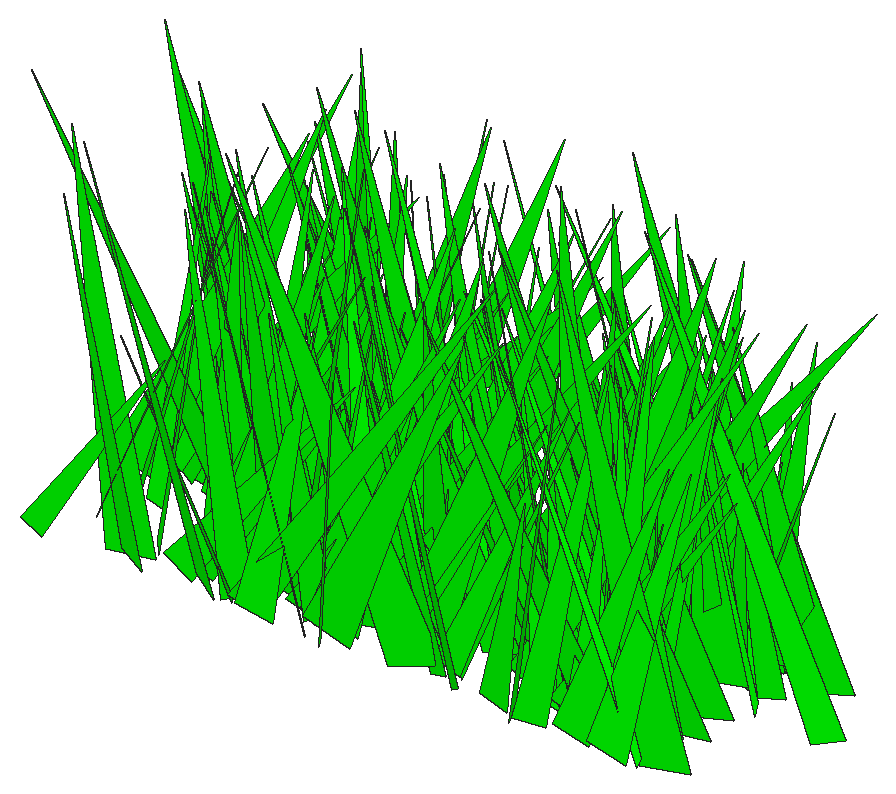
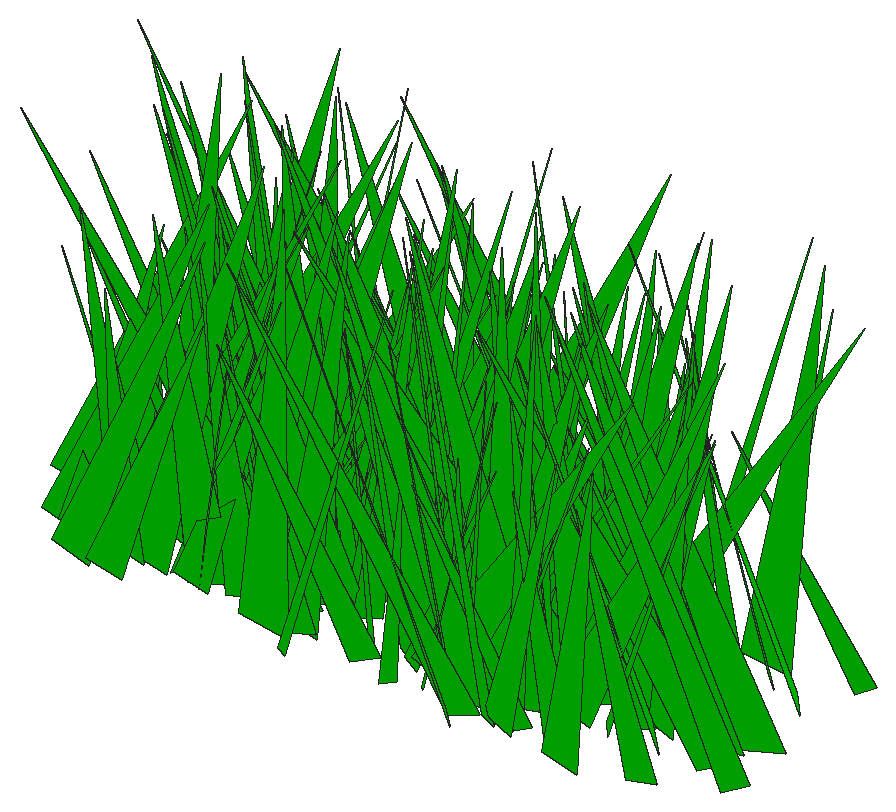
# SketchUp Ruby script. Lengths in inches.
U = 1.inch
M = Sketchup.active_model
def pt(a) = Geom::Point3d.new(a.map { |v| v * U })
def face(e, loops, mat)
  f = e.add_face(loops[0].map { |a| pt(a) })
  loops[1..].each { |l| e.add_face(l.map { |a| pt(a) }).erase! }
  f.material = f.back_material = mat if mat
  f
end
# faces: each face lists its corners as indices into pts; further lists are holes
def faces(e, pts, list, mat = nil) = list.each { |f| face(e, (f[0].is_a?(Array) ? f : [f]).map { |l| l.map { |i| pts[i] } }, mat) }
# xy, xz, yz: faces in a plane at the given z, y or x. An outline is a flat list of corners, or four numbers for a rectangle; further outlines are holes
def ring(l) = l.size == 4 ? [[l[0], l[1]], [l[2], l[1]], [l[2], l[3]], [l[0], l[3]]] : l.each_slice(2).to_a
def flat(e, list, mat, &to3) = list.each { |f| face(e, (f[0].is_a?(Array) ? f : [f]).map { |l| ring(l).map { |u, v| to3.(u, v) } }, mat) }
def xy(e, z, list, mat = nil) = flat(e, list, mat) { |x, y| [x, y, z] }
def xz(e, y, list, mat = nil) = flat(e, list, mat) { |x, z| [x, y, z] }
def yz(e, x, list, mat = nil) = flat(e, list, mat) { |y, z| [x, y, z] }
def lines(e, pts, list) = list.each { |a, b| e.add_line(pt(pts[a]), pt(pts[b])) }
# prism: a flat outline (further loops are holes) pulled along v
def prism(e, loops, v, mat = nil)
  f = face(e, loops, mat); d = Geom::Vector3d.new(v.map { |x| x * U })
  f.pushpull(f.normal.samedirection?(d) ? d.length : -d.length)
end
def box(e, o, s, mat = nil) = prism(e, [[o, [o[0] + s[0], o[1], o[2]], [o[0] + s[0], o[1] + s[1], o[2]], [o[0], o[1] + s[1], o[2]]]], [0, 0, s[2]], mat)
def at(x, y, z, deg = 0) = Geom::Transformation.translation(pt([x, y, z])) * Geom::Transformation.rotation(ORIGIN, Z_AXIS, deg.degrees)
def axes(o, x, y, z) = Geom::Transformation.new([*x, 0, *y, 0, *z, 0, *pt(o).to_a, 1])
def part(name) = M.definitions.add(name)
# library, detail: a bought-in or finely detailed component or shape, given as its bounding box
def library(name, o, s) = part(name).tap { |d| box(d.entities, o, s) }
def detail(e, o, s) = box(e.add_group.entities, o, s)
def put(e, d, t, mat = nil) = e.add_instance(d, t).tap { |i| i.material = mat if mat }
def group(e, t, mat = nil) = e.add_group.tap { |g| g.transformation = t; g.material = mat if mat }.entities
root = M.entities
M.materials.add("[0065_Lime]").color = [0, 255, 0]
c1 = part("fur_instance\#9")
p = [[0.8125,0,1.79],[0.67,-0.02,1.48],[0,-0.11,0],[0,0.11,0]]
faces(c1.entities,p,[[0,1,2,3]])
put(root,c1,axes([68.35,19.12,1.48],[1.92104,-1.04775,2.1483],[7.68559,0.3376,0.9702],[-1.87206,0.31084,6.18757]),"[0065_Lime]")
put(root,c1,axes([69.45,24.6,1.48],[-6.90798,-0.10181,0.94758],[0.97663,-0.95513,1.27214],[0.96343,0.23825,5.50478]),"[0065_Lime]")
put(root,c1,axes([65.31,18.61,1.48],[3.53476,-0.42766,0.80834],[3.08147,0.39799,-1.85976],[0.86889,0.32834,3.30709]),"[0065_Lime]")
put(root,c1,axes([71.52,20.78,1.48],[-6.4799,-0.85162,0.43145],[5.9126,-0.8559,2.14311],[-1.43303,0.31949,6.89142]),"[0065_Lime]")
put(root,c1,axes([68.58,18.88,1.48],[-6.15413,-0.59026,0.7195],[3.89168,-0.85884,-1.58552],[1.81175,-0.16018,5.84974]),"[0065_Lime]")
put(root,c1,axes([64.69,25.02,1.48],[8.06333,-0.48685,0.88652],[3.63083,1.09017,-1.7887],[-0.09462,0.34461,6.91094]),"[0065_Lime]")
put(root,c1,axes([67.125,21.7,1.48],[6.69471,-0.16008,2.11529],[1.84591,0.95655,-1.43968],[-2.15711,0.32173,5.33293]),"[0065_Lime]")
put(root,c1,axes([68.27,23.74,1.48],[6.68983,-0.518,2.03854],[2.93109,0.98966,2.0625],[-3.35842,-0.1681,5.86076]),"[0065_Lime]")
put(root,c1,axes([69.69,23.42,1.48],[2.51525,-1.14828,2.51117],[8.20564,0.4654,1.69312],[-2.99597,0.31066,6.74552]),"[0065_Lime]")
put(root,c1,axes([70.84,24.51,1.48],[-0.91679,0.94632,1.41171],[-6.48248,-0.02719,-2.17456],[-2.51871,-0.27446,5.08288]),"[0065_Lime]")
put(root,c1,axes([66.91,26.29,1.48],[0.68411,-0.6995,0.27313],[4.85295,0.08223,-0.98546],[1.15854,0.06859,3.96665]),"[0065_Lime]")
put(root,c1,axes([69.78,23.02,1.48],[1.5787,0.79457,1.56524],[-5.45357,0.30582,-1.56282],[-2.43637,-0.1697,4.51245]),"[0065_Lime]")
put(root,c1,axes([65.42,22.97,1.48],[1.64409,1.11556,1.21062],[-7.7039,0.15243,2.21546],[2.42736,-0.2718,6.2114]),"[0065_Lime]")
put(root,c1,axes([71.14,24.17,1.48],[-6.88015,0.60712,1.02471],[-4.49889,-0.93646,-1.394],[0.12055,-0.2984,6.4597]),"[0065_Lime]")
put(root,c1,axes([66.4,23.58,1.48],[2.17103,1.16452,0.05617],[-8.14962,0.29815,1.28105],[1.50634,-0.06531,6.84977]),"[0065_Lime]")
put(root,c1,axes([66.27,20.3125,1.48],[8.72768,0.24973,0.46553],[-1.53905,1.17989,-2.11864],[-1.05709,0.34403,6.9282]),"[0065_Lime]")
put(root,c1,axes([68.32,22.84,1.48],[-2.65391,0.63624,0.28444],[-4.09765,-0.36002,1.68903],[1.9578,0.10894,3.92069]),"[0065_Lime]")
put(root,c1,axes([69.28,26.88,1.48],[3.03842,-0.77609,0.00496],[5.27021,0.4077,1.53113],[-1.65206,-0.12678,4.89355]),"[0065_Lime]")
put(root,c1,axes([66.93,23.33,1.48],[6.04871,-0.08994,0.3127],[0.73509,0.7946,-1.74977],[-0.13078,0.30651,4.62782]),"[0065_Lime]")
put(root,c1,axes([71.05,18.95,1.48],[-7.99216,-0.55256,0.60294],[3.62149,-1.09775,-1.9491],[1.7021,-0.25888,6.9781]),"[0065_Lime]")
put(root,c1,axes([67.6,19.81,1.48],[7.73344,0.25591,1.04553],[-1.60675,1.09196,-1.09288],[-1.5451,0.14535,6.36949]),"[0065_Lime]")
put(root,c1,axes([68.67,19.9,1.48],[6.51938,0.05109,1.60015],[-0.98298,0.9025,1.68429],[-1.74236,-0.31801,5.03705]),"[0065_Lime]")
put(root,c1,axes([71.42,22.46,1.48],[-6.31564,0.04592,1.05792],[-0.77244,-0.84383,-1.82383],[1.0962,-0.33006,4.80992]),"[0065_Lime]")
put(root,c1,axes([65.83,24.31,1.48],[2.96567,-0.96311,2.07533],[6.5619,0.17958,-3.41155],[3.22936,0.51956,5.02623]),"[0065_Lime]")
put(root,c1,axes([72.04,18.87,1.48],[-4.76381,-0.07754,0.04405],[0.53477,-0.62519,1.38992],[-0.14635,0.23935,3.64483]),"[0065_Lime]")
put(root,c1,axes([68.16,24.125,1.48],[8.31635,0.34784,0.41406],[-1.83086,0.99882,-3.78665],[-1.7421,0.61082,5.95617]),"[0065_Lime]")
put(root,c1,axes([71.09,22.15,1.48],[4.51504,-0.51168,1.58684],[2.68172,0.67193,2.21171],[-3.14226,-0.16176,4.16766]),"[0065_Lime]")
put(root,c1,axes([69.64,21.49,1.48],[4.00086,-0.84633,0.32961],[5.91729,0.56335,0.94841],[-1.19401,-0.04399,5.80456]),"[0065_Lime]")
put(root,c1,axes([70.95,21.35,1.48],[3.66518,-0.68356,1.26875],[4.55252,0.55943,1.39824],[-2.31767,0.01789,4.75292]),"[0065_Lime]")
put(root,c1,axes([69.84,26.12,1.48],[-1.64757,0.6869,0.50919],[-4.71122,-0.24675,1.06789],[1.44657,-0.02126,4.05788]),"[0065_Lime]")
put(root,c1,axes([68.7,23.97,1.48],[1.69245,-0.55072,0.35965],[3.72898,0.20141,-1.27586],[1.28467,0.1409,3.2296]),"[0065_Lime]")
put(root,c1,axes([72.42,25.84,1.48],[-6.50528,0.12939,0.54173],[-0.73196,-0.89306,1.3321],[0.86931,0.21632,5.17554]),"[0065_Lime]")
put(root,c1,axes([72.18,21.05,1.48],[-1.928,0.8871,0.54164],[-6.2842,-0.25287,-0.92229],[-0.89832,-0.13493,5.28946]),"[0065_Lime]")
put(root,c1,axes([72.48,21.85,1.48],[1.47372,-1.19502,2.04646],[8.45244,0.29776,1.79908],[-2.68522,0.28143,6.78624]),"[0065_Lime]")
put(root,c1,axes([71.92,26.26,1.48],[2.7078,0.70632,1.50407],[-4.70658,0.45276,-1.51826],[-2.55605,-0.08543,4.389]),"[0065_Lime]")
put(root,c1,axes([74.25,23.12,1.48],[-7.71029,-0.19198,0.01805],[1.32148,-1.04311,1.71851],[-0.34759,0.29284,6.13314]),"[0065_Lime]")
put(root,c1,axes([70.29,25.74,1.48],[5.65626,-0.02285,1.46593],[-0.45932,0.78575,1.5831],[-1.75026,-0.28006,4.32196]),"[0065_Lime]")
put(root,c1,axes([70.67,23.84,1.48],[-4.0635,1.0657,0.05312],[-7.21549,-0.54641,2.12905],[2.33658,0.166,6.667]),"[0065_Lime]")
put(root,c1,axes([71.875,25.63,1.48],[-7.92677,0.41326,1.77235],[-2.31868,-1.13207,1.98389],[2.8321,0.22984,6.58486]),"[0065_Lime]")
put(root,c1,axes([73.02,21.12,1.48],[3.16708,1.01763,1.30581],[-6.65811,0.49812,-2.32321],[-3.27003,-0.02862,5.99499]),"[0065_Lime]")
put(root,c1,axes([74.93,25.21,1.48],[-1.93715,1.02369,1.59701],[-6.90012,-0.12514,-2.84992],[-3.05223,-0.36681,5.42919]),"[0065_Lime]")
put(root,c1,axes([72.08,19.09,1.48],[5.66412,-0.74574,1.59581],[4.6379,0.83536,2.18939],[-3.24103,-0.10788,5.9219]),"[0065_Lime]")
put(root,c1,axes([70.9,21.29,1.48],[4.70565,0.94097,0.2014],[-6.54395,0.65444,-1.29456],[-1.4424,0.10071,6.53028]),"[0065_Lime]")
put(root,c1,axes([73.21,24.91,1.48],[0.7733,-0.99854,1.88814],[7.20933,0.18636,1.34888],[-1.97758,0.28891,5.65571]),"[0065_Lime]")
put(root,c1,axes([73.92,24.13,1.48],[-0.82948,0.90279,0.70334],[-6.23358,-0.07745,-1.53302],[-1.77981,-0.1495,5.04143]),"[0065_Lime]")
put(root,c1,axes([73.375,21.93,1.48],[-6.63662,0.35878,2.4086],[-3.5877,-0.88466,-2.12489],[1.5543,-0.51007,5.3796]),"[0065_Lime]")
put(root,c1,axes([70.17,20.52,1.48],[2.20365,-0.8752,0.96249],[6.22186,0.26476,-1.35797],[1.21703,0.23115,5.19958]),"[0065_Lime]")
put(root,c1,axes([73.4,20.22,1.48],[-3.22956,-0.40288,1.22892],[3.22937,-0.42522,0.94396],[0.27204,0.26495,3.3836]),"[0065_Lime]")
put(root,c1,axes([70.5,22.81,1.48],[2.78458,-0.73543,0.99269],[5.31238,0.34749,-1.2331],[0.81222,0.24851,4.66189]),"[0065_Lime]")
put(root,c1,axes([72.08,24.39,1.48],[-6.10707,-0.95814,1.8294],[6.47072,-0.91426,-1.75312],[3.11153,0.02073,7.2364]),"[0065_Lime]")
put(root,c1,axes([72.49,22.64,1.48],[3.89497,-0.04542,1.67144],[0.933,0.58597,-0.90493],[-1.85914,0.19891,3.04759]),"[0065_Lime]")
put(root,c1,axes([72.81,20.125,1.48],[-3.85919,-0.97664,0.18074],[6.82242,-0.53867,-1.15258],[1.34543,-0.06983,6.36294]),"[0065_Lime]")
put(root,c1,axes([69.85,20.31,1.48],[7.09166,-0.00725,0.1791],[0.08684,0.98359,-0.9409],[-0.20881,0.16284,5.69135]),"[0065_Lime]")
put(root,c1,axes([74.8,18.55,1.48],[-7.96327,-0.0877,1.18804],[0.87811,-1.11739,1.13044],[1.32351,0.21371,6.39819]),"[0065_Lime]")
put(root,c1,axes([71.0625,19.99,1.48],[-2.73714,0.97285,2.80938],[-7.05841,-0.52481,1.53971],[3.16863,-0.32869,5.85666]),"[0065_Lime]")
put(root,c1,axes([69.79,19.34,1.48],[2.344,0.71962,0.65141],[-4.64176,0.23644,2.29856],[2.30701,-0.25543,3.96291]),"[0065_Lime]")
put(root,c1,axes([70.42,19.52,1.48],[3.20885,-0.54333,0.04601],[3.61815,0.41819,-1.47822],[1.36487,0.16879,3.81045]),"[0065_Lime]")
put(root,c1,axes([73.93,25.09,1.48],[5.81947,0.34316,2.17539],[-1.40303,0.86932,-2.11183],[-3.33883,0.23281,4.67904]),"[0065_Lime]")
put(root,c1,axes([72.92,24.8,1.48],[6.17735,-0.92749,0.46797],[6.21349,0.84934,2.13916],[-2.30013,-0.19655,7.03546]),"[0065_Lime]")
put(root,c1,axes([75.03,21.83,1.48],[-6.41239,-0.06113,1.05776],[0.69563,-0.89805,1.05112],[1.18168,0.19695,5.12115]),"[0065_Lime]")
put(root,c1,axes([75.84,21.9,1.48],[1.6713,1.02963,1.78556],[-6.87504,0.34061,-2.3237],[-3.35308,-0.18516,5.65442]),"[0065_Lime]")
put(root,c1,axes([71.23,26.01,1.48],[4.84109,-0.31149,0.09209],[2.18752,0.66308,-0.93091],[0.37604,0.15272,4.22976]),"[0065_Lime]")
put(root,c1,axes([74.76,25.95,1.48],[-5.99326,-0.13007,1.05201],[0.62914,-0.84463,-1.12778],[1.4607,-0.16987,4.80214]),"[0065_Lime]")
put(root,c1,axes([74.01,25.25,1.48],[2.41619,0.64562,0.22273],[-4.40619,0.33701,-1.10842],[-1.33073,0.05639,4.0745]),"[0065_Lime]")
put(root,c1,axes([72.25,26.25,1.48],[8.42095,-0.18217,1.4288],[0.81257,1.17441,1.84883],[-2.0263,-0.28611,6.67925]),"[0065_Lime]")
put(root,c1,axes([72.98,18.65,1.48],[-0.76014,0.81306,1.00619],[-5.76627,-0.14108,0.9379],[1.32657,-0.14737,4.65339]),"[0065_Lime]")
put(root,c1,axes([73.04,22.48,1.48],[5.10116,-0.03509,1.1362],[0.5886,0.71875,-1.00475],[-1.29113,0.18904,4.03099]),"[0065_Lime]")
put(root,c1,axes([73.54,22.78,1.48],[-3.90133,0.9385,1.18099],[-6.45272,-0.58319,1.42587],[2.25332,-0.04517,6.1279]),"[0065_Lime]")
put(root,c1,axes([71.72,25.09,1.48],[3.36956,-1.12389,1.40913],[8.11841,0.42588,-1.46241],[1.03154,0.31948,6.9065]),"[0065_Lime]")
put(root,c1,axes([72.75,21.02,1.48],[8.51135,-0.10725,1.91097],[0.28924,1.21953,1.44115],[-2.45321,-0.22832,6.79999]),"[0065_Lime]")
put(root,c1,axes([74.45,19.64,1.48],[5.19055,-0.72051,0.37585],[4.31417,0.65903,2.91454],[-2.80952,-0.31916,5.16982]),"[0065_Lime]")
put(root,c1,axes([75.38,20.78,1.48],[-8.10559,0.63749,0.37834],[-3.84332,-1.0266,3.48463],[2.45508,0.49762,6.70414]),"[0065_Lime]")
put(root,c1,axes([75.8125,25.12,1.48],[-4.13838,-0.29857,0.72975],[2.29959,-0.55408,1.03188],[0.17773,0.2169,3.64057]),"[0065_Lime]")
put(root,c1,axes([73.71,20.6,1.48],[4.94821,0.37136,0.65967],[-2.30438,0.68317,-1.45042],[-1.52703,0.17241,4.32637]),"[0065_Lime]")
put(root,c1,axes([76.86,22.66,1.48],[-3.94021,-1.14059,1.81475],[8.37311,-0.49527,1.59763],[-0.86924,0.39942,7.16333]),"[0065_Lime]")
put(root,c1,axes([73.55,26.11,1.48],[6.49183,0.23494,1.32177],[-1.36535,0.93067,-1.10633],[-1.88994,0.13467,5.33946]),"[0065_Lime]")
put(root,c1,axes([75.39,23.11,1.48],[-4.17587,-0.07624,0.7755],[-0.03028,-0.51908,-1.81781],[1.09653,-0.30466,2.90309]),"[0065_Lime]")
put(root,c1,axes([75.68,19.96,1.48],[1.10215,-0.8776,0.4374],[6.12716,0.16702,1.01424],[-1.32395,0.0424,5.05795]),"[0065_Lime]")
put(root,c1,axes([77.15,22.75,1.48],[-0.02716,1.20622,1.81891],[-8.53852,0.08161,-1.89792],[-2.40432,-0.30346,6.71956]),"[0065_Lime]")
put(root,c1,axes([78.22,19.09,1.48],[-0.03403,-1.22496,2.50395],[8.54875,0.16052,2.70821],[-3.51979,0.4017,6.5534]),"[0065_Lime]")
put(root,c1,axes([76.34,23.95,1.48],[2.51066,-0.75432,1.49569],[5.10828,0.42348,1.48322],[-2.47062,0.10904,4.58665]),"[0065_Lime]")
put(root,c1,axes([72.75,25.75,1.48],[1.33177,1.19653,0.92891],[-8.33656,0.14072,1.83428],[2.07711,-0.20241,6.76635]),"[0065_Lime]")
put(root,c1,axes([76.66,22.3125,1.48],[-0.99939,-0.95897,1.26864],[6.93782,-0.10612,0.92819],[-0.9347,0.23768,5.53307]),"[0065_Lime]")
put(root,c1,axes([73,20.84,1.48],[9.058,0.35471,0.26095],[-2.20962,1.1791,-2.95854],[-1.26196,0.48146,7.0533]),"[0065_Lime]")
put(root,c1,axes([75.66,26.3125,1.48],[-3.44,-0.51784,0.1252],[3.32709,-0.44841,-1.66405],[1.59217,-0.1818,3.74782]),"[0065_Lime]")
put(root,c1,axes([75.34,18.55,1.48],[5.06328,-0.03638,1.54382],[-0.19685,0.73984,1.01141],[-1.9054,-0.17312,3.99797]),"[0065_Lime]")
put(root,c1,axes([74.5,24.6,1.48],[7.76022,-0.05072,1.74355],[-0.18701,1.09697,1.62013],[-2.16563,-0.27649,6.10787]),"[0065_Lime]")
put(root,c1,axes([70.8,23.73,1.48],[4.08989,-1.04553,1.07249],[6.51191,0.38079,-3.99142],[3.8334,0.46862,5.63608]),"[0065_Lime]")
put(root,c1,axes([73.18,26.8,1.48],[8.451,0.00945,0.28621],[-0.21276,1.0716,2.97149],[-0.2882,-0.51411,6.19897]),"[0065_Lime]")
put(root,c1,axes([76.96,23.01,1.48],[-7.04398,-0.43436,1.70674],[2.66579,-1.02522,-1.46357],[2.61753,-0.12478,6.08352]),"[0065_Lime]")
put(root,c1,axes([74.8125,21.61,1.48],[-0.29305,1.03163,1.0635],[-7.19279,-0.08763,1.53697],[1.96808,-0.16664,5.77555]),"[0065_Lime]")
put(root,c1,axes([74.82,19.66,1.48],[-2.81771,1.23234,0.21979],[-8.19191,-0.38377,2.61801],[3.14304,0.10453,7.02054]),"[0065_Lime]")
put(root,c1,axes([78.64,22.48,1.48],[-8.11732,0.44011,1.65121],[-3.46305,-1.14277,-1.05737],[1.39211,-0.27652,6.99776]),"[0065_Lime]")
put(root,c1,axes([73.94,19.57,1.48],[6.55984,0.58092,1.12633],[-4.35749,0.86189,1.89551],[0.14482,-0.38035,6.01554]),"[0065_Lime]")
put(root,c1,axes([76.16,24.82,1.48],[5.62505,0.42866,1.0634],[-2.76904,0.80544,-1.18813],[-1.8296,0.09889,5.0676]),"[0065_Lime]")
put(root,c1,axes([78.45,20.08,1.48],[-6.68093,0.33883,0.32487],[-2.10797,-0.88146,2.12341],[1.23699,0.32786,5.3731]),"[0065_Lime]")
put(root,c1,axes([72.5625,18.82,1.48],[7.64752,-0.71649,0.00096],[4.90952,1.03461,-2.02038],[1.37695,0.29048,7.19834]),"[0065_Lime]")
put(root,c1,axes([72.96,26.41,1.48],[5.4696,0.85102,0.13455],[-5.71976,0.71499,2.30312],[1.99777,-0.2829,6.22561]),"[0065_Lime]")
put(root,c1,axes([75.3125,24.34,1.48],[0.71768,0.83043,1.54257],[-5.95738,0.01691,1.5288],[1.74123,-0.28442,4.59477]),"[0065_Lime]")
put(root,c1,axes([78.97,26.77,1.48],[-7.85854,-0.02685,1.3392],[-0.21681,-1.09474,-1.57735],[1.64321,-0.27287,6.19652]),"[0065_Lime]")
put(root,c1,axes([77.875,20.05,1.48],[-5.41626,0.13666,1.81282],[-1.6622,-0.76617,-1.35039],[1.7748,-0.30049,4.26757]),"[0065_Lime]")
put(root,c1,axes([78.53,21.8,1.48],[-8.40827,0.42582,1.15892],[-2.24502,-1.11833,2.9922],[2.48458,0.43056,6.62572]),"[0065_Lime]")
put(root,c1,axes([73.89,19.62,1.48],[5.92326,-0.65751,0.27557],[4.541,0.78426,-1.87693],[1.17869,0.28278,5.84616]),"[0065_Lime]")
put(root,c1,axes([79,19.09,1.48],[-5.55765,-0.37365,1.25119],[2.95955,-0.77101,0.98257],[0.82327,0.24929,4.91419]),"[0065_Lime]")
put(root,c1,axes([78.46,22.82,1.48],[5.38051,-0.96092,1.92936],[6.36473,0.82588,2.03938],[-3.44678,0.02503,6.77764]),"[0065_Lime]")
put(root,c1,axes([76.95,25.35,1.48],[5.63501,0.12731,1.78635],[-1.46242,0.8119,1.11343],[-1.87217,-0.25104,4.50696]),"[0065_Lime]")
put(root,c1,axes([74.45,21.25,1.48],[6.21251,-0.38772,0.55144],[2.75918,0.76859,-2.45881],[0.67813,0.42475,4.95256]),"[0065_Lime]")
put(root,c1,axes([79.59,21.09,1.48],[-0.19601,-0.83896,1.738],[5.9891,0.07422,1.64743],[-2.08387,0.29222,4.57127]),"[0065_Lime]")
put(root,c1,axes([77.58,20.75,1.48],[-3.93675,-0.11457,2.01894],[1.78083,-0.57919,1.19617],[1.91155,0.30363,3.04354]),"[0065_Lime]")
put(root,c1,axes([78.3,23.875,1.48],[-6.28278,-0.80456,0.59138],[5.32396,-0.86619,-2.06462],[2.22878,-0.1989,6.59889]),"[0065_Lime]")
put(root,c1,axes([79.84,18.75,1.48],[-8.34912,-0.19754,1.50134],[1.75854,-1.17068,1.30903],[1.51344,0.27051,6.76133]),"[0065_Lime]")
put(root,c1,axes([75.17,19.04,1.48],[0.70848,-1.09846,0.21547],[7.36601,0.08113,-2.1659],[2.63088,0.06866,6.00612]),"[0065_Lime]")
put(root,c1,axes([77.85,20.6875,1.48],[-4.63563,-0.9148,0.09538],[6.11381,-0.61848,-2.17266],[2.24015,-0.20508,6.12699]),"[0065_Lime]")
put(root,c1,axes([75.71,22.15,1.48],[-3.32207,1.17858,0.68772],[-7.37563,-0.4682,3.31385],[4.0821,0.11318,6.54721]),"[0065_Lime]")
put(root,c1,axes([79.36,22.9,1.48],[-5.78518,-0.6636,0.31814],[4.27308,-0.76803,-2.2703],[2.04845,-0.272,5.63435]),"[0065_Lime]")
put(root,c1,axes([75.92,22.73,1.48],[4.16429,1.14439,0.96725],[-8.08089,0.53296,1.88935],[1.56185,-0.29374,7.19639]),"[0065_Lime]")
put(root,c1,axes([79.64,25.35,1.48],[4.95435,-0.94797,0.68252],[6.18459,0.68906,2.3668],[-2.82268,-0.15412,6.3837]),"[0065_Lime]")
put(root,c1,axes([81.87,20.4,1.48],[-6.01377,-0.30364,0.29005],[2.17307,-0.80905,1.42972],[-0.27265,0.24909,4.99739]),"[0065_Lime]")
put(root,c1,axes([76.94,25.68,1.48],[3.22137,-0.61978,1.2972],[4.50089,0.33206,-2.07898],[1.31893,0.3806,3.92627]),"[0065_Lime]")
put(root,c1,axes([80.75,22.12,1.48],[-6.36604,0.11536,1.51274],[-1.30643,-0.89033,-1.36255],[1.5575,-0.27531,5.04017]),"[0065_Lime]")
put(root,c1,axes([82.28,22.74,1.48],[-7.22341,0.17943,0.60609],[-1.4479,-0.96412,-1.85323],[0.29881,-0.33421,5.67162]),"[0065_Lime]")
put(root,c1,axes([80.47,21.16,1.48],[2.54223,-0.8567,0.72321],[5.78834,0.3784,1.55775],[-2.11099,0.00586,5.14229]),"[0065_Lime]")
put(root,c1,axes([77.1875,19.84,1.48],[5.98034,0.18227,0.15584],[-1.29932,0.80688,1.36669],[0.1763,-0.23633,4.7863]),"[0065_Lime]")
put(root,c1,axes([81.77,23.96,1.48],[-4.44983,-0.10228,0.06616],[0.70838,-0.58314,1.31508],[-0.18611,0.22596,3.42378]),"[0065_Lime]")
put(root,c1,axes([77.52,20.08,1.48],[2.38314,-1.13329,0.91505],[7.96511,0.29015,-1.68363],[1.6937,0.23009,6.63025]),"[0065_Lime]")
put(root,c1,axes([80.23,25.98,1.48],[4.06245,-1.05842,0.33063],[7.32714,0.5691,1.48076],[-1.79259,-0.07245,6.80184]),"[0065_Lime]")
put(root,c1,axes([79.13,25.63,1.48],[-0.39266,-0.61965,0.23581],[4.15942,-0.06564,-1.19685],[1.49299,0.01989,3.39642]),"[0065_Lime]")
put(root,c1,axes([82.37,21.08,1.48],[-4.17736,-0.31059,0.33227],[2.21322,-0.5472,1.27054],[-0.39247,0.22006,3.62823]),"[0065_Lime]")
put(root,c1,axes([75.8,20.4,1.48],[7.5714,-0.78823,0.26987],[5.31813,0.97989,-2.81672],[1.81476,0.41703,7.12843]),"[0065_Lime]")
put(root,c1,axes([80.3,22.12,1.48],[4.25127,0.55143,0.2746],[-3.55769,0.56755,-1.74774],[-1.69019,0.19236,4.36951]),"[0065_Lime]")
put(root,c1,axes([82.9,22.01,1.48],[-2.83123,-1.14232,1.99744],[8.40409,-0.32464,1.66029],[-1.21986,0.41467,6.80241]),"[0065_Lime]")
put(root,c1,axes([78.89,19.58,1.48],[4.19754,0.62881,0.60972],[-4.52067,0.56731,0.98635],[0.3883,-0.19275,4.89227]),"[0065_Lime]")
put(root,c1,axes([79.27,23.69,1.48],[-0.8762,1.01784,0.3361],[-6.88074,-0.13512,1.84375],[2.30106,-0.01648,5.64127]),"[0065_Lime]")
put(root,c1,axes([81.24,22.75,1.48],[4.81355,-1.10029,1.59575],[7.70587,0.72193,1.30053],[-2.40448,0.11095,7.3625]),"[0065_Lime]")
put(root,c1,axes([82.68,23.72,1.48],[2.47779,-0.96708,1.93125],[6.74545,0.43754,1.61576],[-2.73898,0.2027,5.72631]),"[0065_Lime]")
put(root,c1,axes([84.1875,19.61,1.48],[-3.95382,-0.91251,0.11208],[6.34056,-0.5373,1.40857],[-1.40957,0.14267,6.02171]),"[0065_Lime]")
put(root,c1,axes([79.34,19.61,1.48],[6.28453,0.13492,0.568],[-1.11551,0.852,1.38456],[-0.40646,-0.25214,4.98244]),"[0065_Lime]")
put(root,c1,axes([82.23,19.69,1.48],[-4.94106,0.5475,0.58765],[-3.67461,-0.69377,1.21686],[1.48343,0.10509,4.97164]),"[0065_Lime]")
put(root,c1,axes([79.45,23.78,1.48],[5.86652,-0.61386,1.35486],[4.66649,0.79187,-1.34667],[-0.28715,0.32753,5.79521]),"[0065_Lime]")
put(root,c1,axes([83.84,20.94,1.48],[-1.36101,-0.62916,0.92929],[4.30079,-0.11127,1.64327],[-1.68995,0.22353,3.43358]),"[0065_Lime]")
put(root,c1,axes([83.01,19.77,1.48],[-8.21331,-0.31139,1.70549],[1.90553,-1.18442,-1.17486],[2.38244,-0.12618,6.81925]),"[0065_Lime]")
put(root,c1,axes([81.11,18.82,1.48],[-1.23009,-0.64993,0.30186],[4.42112,-0.18054,-1.10535],[1.40865,-0.0009,3.73279]),"[0065_Lime]")
put(root,c1,axes([83.26,25.32,1.48],[0.03178,-0.78489,0.48806],[5.41055,0.02697,1.22008],[-1.51184,0.08001,4.37665]),"[0065_Lime]")
put(root,c1,axes([83.98,24.88,1.48],[-6.75511,0.33219,0.06972],[-2.23399,-0.90781,1.72538],[0.77797,0.27755,5.55989]),"[0065_Lime]")
put(root,c1,axes([82.33,20.08,1.48],[2.19538,0.67654,0.05734],[-4.59432,0.29757,-1.26357],[-1.44149,0.08195,4.11456]),"[0065_Lime]")
put(root,c1,axes([81.61,25.03,1.48],[-2.82886,0.79532,1.54015],[-5.61941,-0.45412,1.02888],[2.01043,-0.15024,5.04296]),"[0065_Lime]")
put(root,c1,axes([81.65,23.82,1.48],[5.73478,0.3828,0.74791],[-2.15173,0.76261,-2.16293],[-1.90703,0.29068,4.68954]),"[0065_Lime]")
put(root,c1,axes([83.07,25.23,1.48],[-4.42434,-0.02732,1.16357],[0.56101,-0.6296,0.91606],[1.33017,0.17467,3.48387]),"[0065_Lime]")
put(root,c1,axes([84.85,20.48,1.48],[-7.24881,0.1959,0.77457],[-1.53178,-1.01117,-0.91529],[0.70991,-0.18153,5.93416]),"[0065_Lime]")
put(root,c1,axes([81.95,20.91,1.48],[5.09288,0.05622,1.24945],[0.2725,0.68365,-1.76573],[-1.56374,0.30224,3.76157]),"[0065_Lime]")
put(root,c1,axes([81.71,21.91,1.48],[-0.46498,-1.15701,0.38064],[8.15512,-0.07432,-0.97852],[1.2291,0.0554,6.63651]),"[0065_Lime]")
put(root,c1,axes([85.27,25.08,1.48],[-0.74316,1.24548,1.76664],[-8.83495,-0.02151,-1.95084],[-2.28542,-0.32184,6.96705]),"[0065_Lime]")
put(root,c1,axes([85.23,22.35,1.48],[-8.79241,0.00449,1.19286],[0.3804,-1.20245,2.00668],[1.41665,0.35072,6.86462]),"[0065_Lime]")
put(root,c1,axes([81.81,18.76,1.48],[7.84133,-0.16411,1.56782],[0.2694,1.04173,2.76228],[-2.23751,-0.44968,5.82702]),"[0065_Lime]")
put(root,c1,axes([84.82,23.64,1.48],[-5.55467,-0.52218,1.39978],[4.06266,-0.75392,1.24252],[0.51536,0.31512,5.29221]),"[0065_Lime]")
put(root,c1,axes([86.52,23.83,1.48],[-9.12482,0.21766,0.58579],[-1.68386,-1.23863,-1.93255],[0.28739,-0.3465,7.27616]),"[0065_Lime]")
put(root,c1,axes([86.43,20.68,1.48],[-5.1978,-1.02539,0.3671],[7.22661,-0.70876,1.36229],[-1.10862,0.18745,7.15903]),"[0065_Lime]")
put(root,c1,axes([82.79,25.02,1.48],[-3.19631,1.05353,0.08757],[-7.19684,-0.43565,1.82507],[2.10475,0.11028,6.3735]),"[0065_Lime]")
put(root,c1,axes([81.32,22.2,1.48],[-0.80437,1.23555,1.57932],[-8.56665,-0.18939,2.07805],[2.7742,-0.22659,6.87487]),"[0065_Lime]")
put(root,c1,axes([84.94,20.93,1.48],[-1.50007,-0.60821,0.81196],[4.36344,-0.17404,0.96515],[-0.83172,0.18389,3.59904]),"[0065_Lime]")
put(root,c1,axes([82.55,18.56,1.48],[5.01015,0.85529,0.11124],[-5.99096,0.69702,-1.05157],[-1.08402,0.10083,6.32573]),"[0065_Lime]")
put(root,c1,axes([84.09,22.22,1.48],[4.35103,-0.64434,0.61989],[3.92865,0.58814,2.24038],[-2.4846,-0.19841,4.62803]),"[0065_Lime]")
put(root,c1,axes([85.59,26.18,1.48],[-2.0129,0.78284,0.70787],[-5.52107,-0.24725,-1.22511],[-1.14571,-0.18392,4.66]),"[0065_Lime]")
put(root,c1,axes([83.58,19.41,1.48],[-2.13929,0.60123,0.54466],[-4.13116,-0.3148,0.90821],[1.29958,-0.01099,3.78364]),"[0065_Lime]")
put(root,c1,axes([86.18,18.85,1.48],[-7.55741,-0.012,0.7713],[-0.18637,-1.02676,-1.74347],[0.93364,-0.30208,5.89528]),"[0065_Lime]")
put(root,c1,axes([81.82,22.77,1.48],[-1.12564,-1.17455,0.31844],[7.85348,-0.16745,-2.32813],[2.88877,-0.00245,6.45339]),"[0065_Lime]")
put(root,c1,axes([83.2,20.41,1.48],[7.02258,0.45956,1.53315],[-3.0545,1.02051,-0.9933],[-2.21785,0.04967,6.22256]),"[0065_Lime]")
put(root,c1,axes([80.74,24.61,1.48],[5.15532,-0.85589,0.4651],[5.94817,0.67668,-1.89595],[1.43041,0.27079,6.2078]),"[0065_Lime]")
put(root,c1,axes([84.14,21.95,1.48],[-5.87993,0.65707,0.61157],[-3.91888,-0.76957,2.77668],[2.65955,0.31873,5.44357]),"[0065_Lime]")
put(root,c1,axes([82.24,22.6,1.48],[7.9062,-0.22655,1.5906],[2.08079,1.09414,-1.62107],[-1.44692,0.33554,6.36002]),"[0065_Lime]")
put(root,c1,axes([86.3,21.86,1.48],[-0.57932,-0.916,0.70759],[6.27969,-0.0406,1.64066],[-1.9535,0.14114,5.06419]),"[0065_Lime]")
put(root,c1,axes([83.7,23.04,1.48],[-3.34143,0.69014,1.46325],[-4.73231,-0.52666,1.17344],[2.22783,-0.0836,4.68727]),"[0065_Lime]")
put(root,c1,axes([84.74,19.82,1.48],[-4.49012,0.70595,0.68102],[-4.79333,-0.63874,1.27669],[1.72184,0.0628,5.33003]),"[0065_Lime]")
put(root,c1,axes([84.04,19.65,1.48],[4.57521,-0.12503,1.06713],[0.31542,0.62364,1.55373],[-1.5535,-0.24161,3.45827]),"[0065_Lime]")
put(root,c1,axes([85.8,20.24,1.48],[2.02227,0.96664,1.56758],[-6.77891,0.34847,-1.41422],[-2.25455,-0.1807,5.65831]),"[0065_Lime]")
put(root,c1,axes([86.86,26.03,1.48],[-3.61225,-0.87311,1.14215],[6.30932,-0.45908,1.443],[-0.87879,0.29295,5.66532]),"[0065_Lime]")
put(root,c1,axes([79.86,24.72,1.48],[5.45079,1.03002,0.39149],[-6.74198,0.668,3.2149],[2.91708,-0.38079,6.69879]),"[0065_Lime]")
put(root,c1,axes([85.26,23.52,1.48],[3.91714,-1.14093,1.79905],[8.06875,0.60657,1.2662],[-2.39019,0.17785,7.22276]),"[0065_Lime]")
put(root,c1,axes([84.99,21.02,1.48],[-4.18637,-0.1203,1.73061],[1.48277,-0.61669,0.93669],[1.74958,0.23478,3.34713]),"[0065_Lime]")
put(root,c1,axes([82.54,22.16,1.48],[3.76759,-0.93669,1.51544],[6.86617,0.46819,-1.59722],[0.87329,0.36001,6.02007]),"[0065_Lime]")
put(root,c1,axes([80.9,20.35,1.48],[7.72902,0.73751,0.01687],[-5.16281,1.06738,1.39237],[0.94477,-0.2006,7.47076]),"[0065_Lime]")
put(root,c1,axes([86.39,25.16,1.48],[-3.95485,-0.33713,0.72372],[2.55626,-0.5309,0.95532],[0.11545,0.20641,3.6393]),"[0065_Lime]")
put(root,c1,axes([85.1,23.65,1.48],[2.76661,-0.59142,0.02306],[3.97947,0.3691,1.32008],[-1.37091,-0.12211,3.87847]),"[0065_Lime]")
put(root,c1,axes([82.35,24.53,1.48],[5.00724,0.60722,0.28451],[-4.27639,0.67942,1.20716],[0.71292,-0.18939,5.24279]),"[0065_Lime]")
put(root,c1,axes([87.05,18.83,1.48],[1.57964,1.16792,2.51961],[-8.3647,0.34323,-1.86148],[-2.95098,-0.34773,6.62518]),"[0065_Lime]")
put(root,c1,axes([82.6,21.3,1.48],[4.05339,-0.48011,0.02526],[3.2755,0.54405,-1.25635],[0.97278,0.16864,4.1251]),"[0065_Lime]")
put(root,c1,axes([84.6,19.69,1.48],[4.5759,0.17869,0.76586],[-0.60156,0.57091,-2.08552],[-1.46349,0.32406,3.25186]),"[0065_Lime]")
put(root,c1,axes([82.97,21.83,1.48],[2.64163,-1.10601,1.84237],[8.0747,0.29567,-1.71258],[1.37185,0.38944,6.53258]),"[0065_Lime]")
put(root,c1,axes([84.94,24.83,1.48],[-2.73728,0.51396,0.16006],[-3.25064,-0.35676,1.60573],[1.68828,0.14639,3.35122]),"[0065_Lime]")
put(root,c1,axes([87.94,24.88,1.48],[-1.39943,1.03208,1.84242],[-7.36104,-0.08687,-2.06877],[-2.21184,-0.3639,5.71921]),"[0065_Lime]")
put(root,c1,axes([84.79,19.09,1.48],[5.82573,-0.5961,3.10437],[5.37224,0.83132,-1.32137],[-1.92372,0.51637,5.71109]),"[0065_Lime]")
put(root,c1,axes([83.86,18.74,1.48],[-1.3193,0.75698,2.01041],[-5.40614,-0.29954,1.43198],[2.42954,-0.25546,4.2781]),"[0065_Lime]")
put(root,c1,axes([85.54,25.17,1.48],[2.6093,0.743,0.04824],[-5.18404,0.36126,-0.92256],[-1.04289,0.0632,4.70659]),"[0065_Lime]")
put(root,c1,axes([85.42,23.9,1.48],[-2.5931,-0.61122,0.31928],[4.06131,-0.36106,-1.33706],[1.60626,-0.07382,3.89611]),"[0065_Lime]")
put(root,c1,axes([82.98,19.73,1.48],[2.78474,-0.83457,0.78363],[5.69333,0.31723,-2.06529],[1.94646,0.2661,4.91981]),"[0065_Lime]")
put(root,c1,axes([84.88,21.12,1.48],[6.60499,-0.13042,1.77657],[1.4482,0.94057,-1.24859],[-1.88001,0.26632,5.27974]),"[0065_Lime]")
put(root,c1,axes([86.85,23.6875,1.48],[1.39718,0.66684,0.40272],[-4.46125,0.20829,-1.3161],[-1.69202,0.00147,3.80263]),"[0065_Lime]")
put(root,c1,axes([86.9,22.95,1.48],[-5.90034,-0.0821,1.23108],[0.06289,-0.81315,-1.61766],[1.62112,-0.26727,4.5435]),"[0065_Lime]")
put(root,c1,axes([87.43,24.96,1.48],[1.71007,-0.84633,1.85702],[6.01692,0.32836,1.34851],[-2.29882,0.22986,4.911]),"[0065_Lime]")
put(root,c1,axes([85.49,25.08,1.48],[-2.8074,0.78442,1.7841],[-5.60256,-0.46446,1.00979],[2.14122,-0.18679,4.98132]),"[0065_Lime]")
put(root,c1,axes([85.24,18.55,1.48],[-0.92507,0.8981,0.04492],[-6.16126,-0.12739,1.39132],[1.70052,0.02702,5.06541]),"[0065_Lime]")
put(root,c1,axes([89.55,22.75,1.48],[-7.93984,0.61159,1.104],[-4.55741,-1.07521,-1.72678],[0.12514,-0.35362,7.15979]),"[0065_Lime]")
put(root,c1,axes([84.95,24.65,1.48],[5.70909,0.05155,0.6842],[-0.1649,0.79028,-1.08483],[-0.90273,0.18166,4.52521]),"[0065_Lime]")
